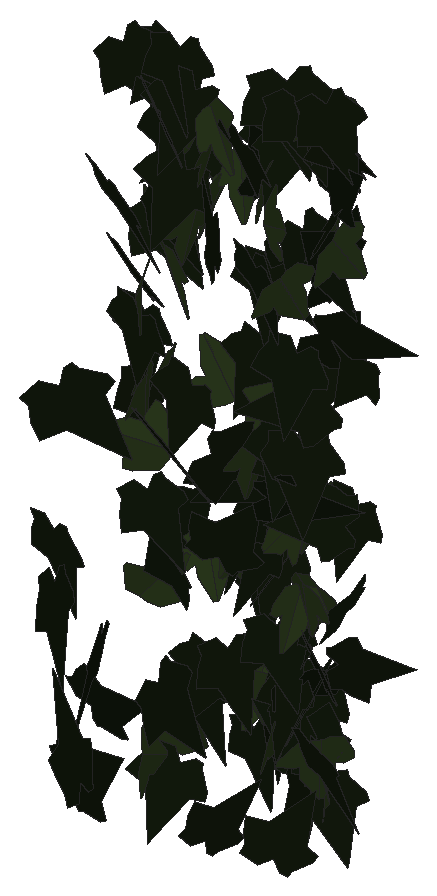
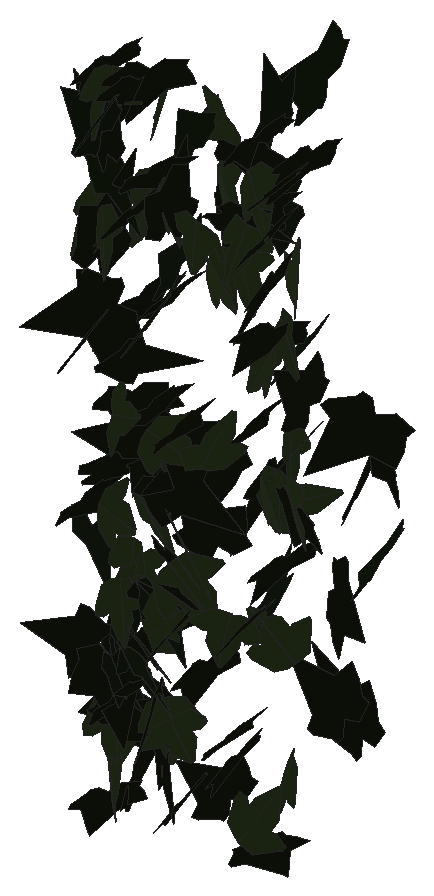
# SketchUp Ruby script. Lengths in inches.
U = 1.inch
M = Sketchup.active_model
def pt(a) = Geom::Point3d.new(a.map { |v| v * U })
def face(e, loops, mat)
  f = e.add_face(loops[0].map { |a| pt(a) })
  loops[1..].each { |l| e.add_face(l.map { |a| pt(a) }).erase! }
  f.material = f.back_material = mat if mat
  f
end
# faces: each face lists its corners as indices into pts; further lists are holes
def faces(e, pts, list, mat = nil) = list.each { |f| face(e, (f[0].is_a?(Array) ? f : [f]).map { |l| l.map { |i| pts[i] } }, mat) }
# xy, xz, yz: faces in a plane at the given z, y or x. An outline is a flat list of corners, or four numbers for a rectangle; further outlines are holes
def ring(l) = l.size == 4 ? [[l[0], l[1]], [l[2], l[1]], [l[2], l[3]], [l[0], l[3]]] : l.each_slice(2).to_a
def flat(e, list, mat, &to3) = list.each { |f| face(e, (f[0].is_a?(Array) ? f : [f]).map { |l| ring(l).map { |u, v| to3.(u, v) } }, mat) }
def xy(e, z, list, mat = nil) = flat(e, list, mat) { |x, y| [x, y, z] }
def xz(e, y, list, mat = nil) = flat(e, list, mat) { |x, z| [x, y, z] }
def yz(e, x, list, mat = nil) = flat(e, list, mat) { |y, z| [x, y, z] }
def lines(e, pts, list) = list.each { |a, b| e.add_line(pt(pts[a]), pt(pts[b])) }
# prism: a flat outline (further loops are holes) pulled along v
def prism(e, loops, v, mat = nil)
  f = face(e, loops, mat); d = Geom::Vector3d.new(v.map { |x| x * U })
  f.pushpull(f.normal.samedirection?(d) ? d.length : -d.length)
end
def box(e, o, s, mat = nil) = prism(e, [[o, [o[0] + s[0], o[1], o[2]], [o[0] + s[0], o[1] + s[1], o[2]], [o[0], o[1] + s[1], o[2]]]], [0, 0, s[2]], mat)
def at(x, y, z, deg = 0) = Geom::Transformation.translation(pt([x, y, z])) * Geom::Transformation.rotation(ORIGIN, Z_AXIS, deg.degrees)
def axes(o, x, y, z) = Geom::Transformation.new([*x, 0, *y, 0, *z, 0, *pt(o).to_a, 1])
def part(name) = M.definitions.add(name)
# library, detail: a bought-in or finely detailed component or shape, given as its bounding box
def library(name, o, s) = part(name).tap { |d| box(d.entities, o, s) }
def detail(e, o, s) = box(e.add_group.entities, o, s)
def put(e, d, t, mat = nil) = e.add_instance(d, t).tap { |i| i.material = mat if mat }
def group(e, t, mat = nil) = e.add_group.tap { |g| g.transformation = t; g.material = mat if mat }.entities
root = M.entities
M.materials.add("efeu1").color = [18, 25, 13]
M.materials.add("efeu2").color = [43, 57, 29]
c1 = part("ivyleaf_9")
p = [[1.54,2.16,1.25],[1.36,2.04,1.19],[-0.21,0.99,0.68],[-0.71,1.11,0.82],[-0.85,0.86,0.67],[-0.8,0.17,0.21],
  [-0.9,-0.01,0.1],[-0.67,-0.16,-0.02],[-0.08,-0.08,-0.05],[-0.03,-0.6,-0.4],[0.65,-0.88,-0.66],[0.83,-0.6,-0.49],
  [1.29,-0.42,-0.43],[1.8125,-0.07,-0.26],[1.21,0.44,0.15]]
faces(c1.entities,p,[[0,1,2,3,4,5,6,7,8,9,10,11,12,13,14]],"efeu1")
c2 = part("ivyleaf_10")
p = [[0,0.5,-0.03],[-0.0625,2.02,-0.43],[-0.19,2.01,-0.46],[-0.54,1.05,-0.29],[-0.52,0.625,-0.18],[-0.83,0.76,-0.28],
  [-1.16,0.64,-0.33],[-1.15,0.33,-0.24],[-0.77,-0.39,0.02],[-0.3,-0.51,0.16],[0.04,-0.48,0.23],[-0.02,2.01,-0.4375],
  [-0.06,2.01,-0.43],[0.04,-0.49,0.23],[0.67,-0.49,0.14],[1.38,0.36,-0.2],[1.375,0.51,-0.24],[0.81,0.65,-0.19],
  [0.62,0.59,-0.15],[0.6,1.09,-0.28],[0.5,1.23,-0.31]]
faces(c2.entities,p,[[0,1,2,3,4,5,6,7,8,9,10],[11,12,0,13,14,15,16,17,18,19,20]],"efeu2")
put(root,c1,axes([573.86,110.85,251.43],[-0.10242,-1.0928,1.02253],[0.0901,1.01856,1.09759],[-1.49388,0.13636,-0.00391]))
put(root,c1,axes([569.65,114.63,256.8],[-0.54052,-0.11963,-1.31812],[1.32353,-0.04442,-0.53871],[0.00412,-1.42395,0.12754]))
put(root,c1,axes([574.41,114.41,265.84],[1.30871,-0.42606,-0.11403],[-0.10734,0.03865,-1.37631],[0.42779,1.3131,0.00351]))
put(root,c1,axes([574.72,114.92,254.02],[0.53059,-0.75779,-0.98755],[-0.56809,0.80779,-0.92508],[1.10759,0.77733,-0.00139]))
put(root,c1,axes([570.54,117,273.96],[0.85935,-1.02214,0.66736],[0.41204,-0.52536,-1.33523],[1.14907,0.95281,-0.0203]))
put(root,c1,axes([567.85,118.16,245.98],[-0.09268,0.13273,1.43159],[0.9184,-1.09826,0.16129],[1.10617,0.92296,-0.01396]))
put(root,c1,axes([568.71,118.59,252.28],[-0.60556,0.38599,-1.26243],[1.0818,-0.65093,-0.71794],[-0.7566,-1.23965,-0.0161]))
put(root,c1,axes([565.42,119.9375,255.38],[0.49386,-1.12594,0.3271],[0.11112,-0.30839,-1.2293],[1.16722,0.50575,-0.02137]))
put(root,c1,axes([566.99,120.38,248.06],[0.15052,-0.24375,1.19736],[0.96166,-0.72066,-0.26759],[0.75386,0.96797,0.10228]))
put(root,c2,axes([568.71,121.3,266.89],[0.16425,-0.42355,-1.17811],[0.38377,-1.11397,0.454],[-1.19166,-0.41712,-0.01618]))
put(root,c1,axes([565.63,120.14,261.83],[-0.18279,-0.35002,-1.29683],[0.53968,1.17936,-0.39438],[1.23005,-0.56946,-0.01967]))
put(root,c2,axes([576.26,119.86,272.95],[-0.41112,0.4522,0.99052],[-0.61499,0.77729,-0.61011],[-0.89856,-0.7389,-0.03562]))
put(root,c1,axes([569.27,121.72,274.38],[0.04519,-0.46985,1.26714],[0.48066,-1.17936,-0.45444],[1.26308,0.46561,0.1276]))
put(root,c1,axes([575.69,120.79,244.23],[-0.56694,-0.08051,0.91684],[0.91933,0.00165,0.56862],[-0.04375,1.07797,0.06761]))
put(root,c1,axes([567.74,122.29,264.79],[0.10552,-1.03428,0.57558],[0.15766,-0.56044,-1.03596],[1.17311,0.16835,0.08745]))
put(root,c2,axes([575.56,121.5,269.35],[-0.42794,-0.97958,-0.5903],[0.21639,0.54954,-1.0688],[1.12303,-0.47916,-0.01899]))
put(root,c1,axes([571.68,121.63,243.26],[-0.10455,-0.20583,1.03103],[0.91019,0.5009,0.19229],[-0.52625,0.90722,0.12775]))
put(root,c1,axes([574.98,123.03,265.28],[-0.17149,-1.15961,0.09107],[-0.02017,-0.08908,-1.17221],[1.16301,-0.17254,-0.0069]))
put(root,c1,axes([571.78,121.875,269.02],[0.01584,-0.13978,1.28616],[-0.33463,1.24204,0.1391],[-1.2497,-0.33435,-0.02095]))
put(root,c2,axes([568.38,121.85,245.76],[0.28146,-0.57133,-1.07538],[-0.04694,1.09782,-0.59554],[1.21682,0.1745,0.22578]))
put(root,c2,axes([570.93,122.84,274.54],[0.74797,-0.10302,0.86127],[0.85496,-0.1045,-0.75498],[0.14649,1.13593,0.00866]))
put(root,c1,axes([569.05,123.47,271.24],[-0.42757,-1.09553,0.2771],[-0.08596,-0.26388,-1.17591],[1.12675,-0.43585,0.01544]))
put(root,c1,axes([568.19,123.6,253.67],[0.8151,-0.70151,-0.67063],[0.50656,-0.43949,1.07541],[-0.8278,-0.95968,-0.00226]))
put(root,c1,axes([571.42,122.73,255.33],[-0.47971,-0.1477,1.03329],[1.01018,-0.352,0.41866],[0.26279,1.08347,0.27687]))
put(root,c1,axes([571.84,123.63,273.36],[0.20991,-0.86177,0.88202],[0.43517,-0.78537,-0.87091],[1.15379,0.453,0.16801]))
put(root,c1,axes([569.1875,123.71,261.54],[-0.14884,-1.04741,0.50626],[0.001,-0.5105,-1.05589],[1.16334,-0.13356,0.06568]))
put(root,c2,axes([567.65,123.48,258.55],[0.27169,0.35664,1.17355],[-0.7659,-0.88952,0.44764],[0.95802,-0.81227,0.02506]))
put(root,c1,axes([574.03,123.66,260.89],[-0.18133,-1.13237,0.18259],[0.00393,-0.18547,-1.14632],[1.14699,-0.17838,0.03279]))
put(root,c1,axes([572.43,123.71,267.93],[0.47036,-1.01293,0.6329],[0.27772,-0.56881,-1.11676],[1.16166,0.54612,0.01073]))
put(root,c1,axes([575.05,123.39,261.03],[-0.54185,-0.95578,-0.49638],[0.20934,0.4516,-1.09807],[1.05645,-0.5797,-0.03701]))
put(root,c2,axes([567.47,122.92,261.53],[0.25977,-1.00547,-0.38903],[-0.01331,0.39714,-1.03533],[1.07803,0.24719,0.08096]))
put(root,c1,axes([573.98,122.7,258.71],[0.53554,0.54877,-1.05958],[0.72953,0.76849,0.76673],[0.94427,-0.90495,0.00857]))
put(root,c1,axes([575.41,123.5,247.73],[0.87827,-0.96416,0.25234],[0.15994,-0.19563,-1.30414],[0.98372,0.89262,-0.01325]))
put(root,c1,axes([567.32,123.42,256.34],[0.27879,-1.02264,-0.48464],[0.0414,0.50801,-1.04814],[1.13091,0.23351,0.15784]))
put(root,c2,axes([572.5625,123.64,260.12],[-0.0623,-1.19015,0.11543],[0.01415,-0.11631,-1.19161],[1.19565,-0.06064,0.02012]))
put(root,c2,axes([567.41,123.36,252.11],[-0.6393,-0.65848,0.65321],[0.46375,0.46012,0.91772],[-0.80325,0.78973,0.00996]))
put(root,c1,axes([571.07,123.69,250.41],[0.13657,-1.03082,-0.47157],[-0.092,0.46334,-1.03946],[1.12982,0.16234,-0.02764]))
put(root,c1,axes([575.51,124.1875,262.83],[-0.74346,-0.22338,0.9482],[-0.91351,-0.25443,-0.7762],[0.33836,-1.17775,-0.01216]))
put(root,c1,axes([571.19,122.68,259.72],[0.09394,0.19429,-1.26731],[-0.0812,1.26906,0.18854],[1.27955,0.06627,0.10501]))
put(root,c1,axes([568.97,124.12,274.48],[-1.00288,-0.57528,-0.28926],[0.24598,0.15249,-1.15613],[0.59507,-1.03257,-0.00959]))
put(root,c2,axes([569.18,123.85,269.16],[-0.02815,-1.12054,0.09049],[0.01426,-0.09087,-1.12077],[1.12409,-0.02691,0.01648]))
put(root,c1,axes([576.13,124.4375,257.51],[-0.64533,-0.05727,0.86038],[-0.72474,-0.54624,-0.57996],[0.4672,-0.92646,0.28876]))
put(root,c2,axes([574.29,124.05,253.76],[0.38268,0.90143,-0.42788],[-0.20699,-0.37659,-0.97849],[-0.97613,0.43326,0.03974]))
put(root,c1,axes([573.94,124.74,244.86],[0.24506,-0.3699,-1.06214],[0.84467,-0.65725,0.42378],[-0.74263,-0.86961,0.1315]))
put(root,c2,axes([569.88,124.12,272.83],[0.51281,-1.06387,0.03588],[0.00907,-0.03545,-1.18099],[1.06443,0.51284,-0.00722]))
put(root,c1,axes([575.7,124.06,276.17],[0.25693,-1.07445,-0.4585],[0.00744,0.47096,-1.09947],[1.16817,0.23332,0.10785]))
put(root,c1,axes([573.64,124.16,276.4],[-0.26043,-1.07272,-0.67278],[0.2523,0.62913,-1.10079],[1.24085,-0.35306,0.08262]))
put(root,c1,axes([576.21,123.93,271.5],[-0.8032,0.90095,-0.27324],[0.18572,-0.20049,-1.20699],[-0.92297,-0.82438,-0.00508]))
put(root,c1,axes([575.61,124.41,272.27],[-0.08914,0.04422,1.22627],[0.68922,-1.01542,0.08671],[1.01521,0.69324,0.0488]))
put(root,c1,axes([577.01,123.49,254.33],[-0.37109,0.9234,0.4039],[-0.18332,0.36138,-0.99464],[-0.99106,-0.41261,0.03275]))
put(root,c1,axes([567.77,124.65,243.75],[-0.59687,-0.94572,0.0103],[0.00597,-0.01595,-1.11824],[0.94576,-0.59674,0.01356]))
put(root,c2,axes([574.8,123.92,254.26],[-0.98483,0.37039,0.21185],[-0.212,0.03772,-1.05147],[-0.3703,-1.00665,0.03855]))
put(root,c1,axes([574.11,124.23,275.76],[0.01345,-1.01618,-0.58211],[0.09864,0.58106,-1.01208],[1.16694,-0.0374,0.09226]))
put(root,c1,axes([573.42,124.59,249.38],[-0.73409,-0.39739,-0.63975],[0.68526,0.01816,-0.7976],[0.31242,-0.97357,0.24625]))
put(root,c1,axes([572.92,124.43,251.75],[0.03625,-1.08694,-0.38663],[0.09147,0.38831,-1.08309],[1.15003,0.00337,0.09833]))
put(root,c2,axes([573.77,124.16,256.93],[0.8255,-0.44156,-0.64322],[-0.57974,0.27952,-0.93591],[0.52213,1.00849,-0.02223]))
put(root,c1,axes([565.63,124.07,275.4375],[0.34713,-0.861,-0.7275],[-0.06637,0.74428,-0.91253],[1.12524,0.30951,0.1706]))
put(root,c2,axes([575.17,124.27,247.24],[-0.74683,-0.98188,-0.02551],[0.01635,0.01961,-1.23363],[0.98208,-0.747,0.00114]))
put(root,c1,axes([572.34,124.7,258.67],[0.01461,-0.01696,-1.27934],[-0.7707,-1.02137,0.00473],[-1.02128,0.77053,-0.02188]))
put(root,c1,axes([567.8,124.72,275.67],[0.05963,-1.16155,-0.10993],[-0.00635,0.10975,-1.16308],[1.16672,0.05996,-0.00071]))
put(root,c2,axes([573.0625,123.91,247.6875],[0.43446,-0.91011,-0.76698],[-0.20039,0.74889,-1.00216],[1.1732,0.46495,0.11286]))
put(root,c1,axes([567.43,124.18,269.29],[0.62539,-0.87453,-0.61668],[-0.36027,0.50051,-1.07513],[1.00762,0.72174,-0.00166]))
put(root,c1,axes([572.28,124.69,255.37],[-1.0218,0.00735,-0.47474],[0.4745,-0.02459,-1.02164],[-0.01703,-1.12643,0.01921]))
put(root,c1,axes([568.95,125.25,248.43],[-0.28575,-0.962,0.52983],[0.03272,-0.55469,-0.98948],[1.09777,-0.23387,0.16741]))
put(root,c1,axes([572.05,125.09,267.15],[-0.07335,-1.08728,0.2572],[0.11437,-0.26371,-1.08217],[1.11142,-0.04462,0.12833]))
put(root,c1,axes([574.76,124.59,246.8],[-0.04284,0.23918,1.108],[-1.12702,0.10964,-0.06724],[-0.12128,-1.1034,0.23349]))
put(root,c1,axes([575.26,125.28,268.21],[0.21824,0.42013,1.3969],[-0.69211,-1.21352,0.4731],[1.28407,-0.72549,0.01758]))
put(root,c1,axes([574.33,124.42,269.93],[0.66415,-1.04697,-0.59352],[-0.16931,0.58987,-1.23],[1.19153,0.6674,0.15605]))
put(root,c1,axes([571.58,124.92,256.62],[-1.04282,0.24053,-0.72523],[0.70936,-0.15119,-1.07015],[-0.28392,-1.26118,-0.01002]))
put(root,c1,axes([574.99,124.7,250.06],[0.38323,-0.84721,0.88138],[-0.39535,0.78816,0.9295],[-1.15685,-0.55001,-0.02568]))
put(root,c1,axes([568.68,124.87,247.63],[0.41567,-1.03663,-0.23213],[-0.08862,0.21457,-1.11686],[1.0586,0.425,-0.00235]))
put(root,c1,axes([564.86,125.17,264.94],[0.42263,-0.62187,0.88306],[0.56717,-0.6792,-0.74976],[0.91914,0.70505,0.05661]))
put(root,c1,axes([568.83,125.3125,272.1],[-1.00169,-0.40724,0.33238],[-0.28176,-0.1879,-1.07935],[0.44377,-1.03853,0.06495]))
put(root,c2,axes([567.27,124.8,266.11],[-0.82288,0.68314,-0.46626],[0.35211,-0.3058,-1.06945],[-0.7484,-0.895,0.00951]))
put(root,c1,axes([565.5625,125.09,259.95],[-0.65793,-0.17528,-0.89599],[0.89176,0.11328,-0.67699],[0.19564,-1.10582,0.07267]))
put(root,c2,axes([575.96,124.35,269.97],[-0.14596,-0.98591,-0.71835],[0.32149,0.66681,-0.98049],[1.17673,-0.30446,0.17877]))
put(root,c1,axes([574.65,125.09,249.99],[-0.79662,0.56117,-0.67503],[0.51945,-0.43348,-0.97337],[-0.70764,-0.94993,0.0454]))
put(root,c1,axes([566.9,125.53,271.7],[0.05803,-1.11771,0.36298],[0.05768,-0.36028,-1.1186],[1.17376,0.07296,0.03703]))
put(root,c1,axes([575.35,125.77,273.69],[-0.37791,-0.39798,1.02082],[-0.1718,-1.04495,-0.47099],[1.0821,-0.30489,0.28173]))
put(root,c2,axes([572.01,125.13,271.67],[0.48291,-1.0045,0.19161],[0.08156,-0.17339,-1.11455],[1.01935,0.48974,-0.00159]))
put(root,c2,axes([575.24,124.59,275.52],[-0.43895,-0.96935,-0.44434],[0.17515,0.40845,-1.06408],[1.05186,-0.47253,-0.00825]))
put(root,c2,axes([572.01,125.66,261.09],[-0.35559,-0.66207,0.84033],[-0.11336,-0.85723,-0.72336],[1.06379,-0.31266,0.20381]))
put(root,c2,axes([567.85,125.16,244.69],[-0.97559,0.00171,-0.57933],[-0.57857,-0.06107,0.97413],[-0.02972,1.13299,0.05338]))
put(root,c2,axes([571.1,125.46,255.06],[-0.54873,-0.88,0.71355],[-0.38531,-0.60063,-1.03704],[1.06541,-0.67046,-0.00754]))
put(root,c1,axes([575.06,125.5,273.82],[0.36367,-0.56307,0.97952],[0.66033,-0.72904,-0.66425],[0.91677,0.74848,0.08988]))
put(root,c1,axes([565.3,125.63,262.67],[0.1953,-1.08259,0.29529],[0.08669,-0.28428,-1.09955],[1.11879,0.21101,0.03365]))
put(root,c2,axes([568.26,124.7,271.49],[-0.25024,-0.9226,-0.63681],[0.21687,0.60032,-0.95495],[1.09986,-0.32828,0.04341]))
put(root,c2,axes([567.43,125.32,273.93],[0.14361,-1.16815,0.11398],[0.01736,-0.11271,-1.17694],[1.17357,0.14461,0.00347]))
put(root,c2,axes([566.48,124.77,267.44],[-0.4563,0.15198,1.0031],[-0.94617,0.33321,-0.48089],[-0.36616,-1.05043,-0.00742]))
put(root,c2,axes([571.85,125.19,248.67],[-0.8731,-0.55762,0.13382],[-0.10318,-0.08703,-1.03583],[0.5641,-0.879,0.01767]))
put(root,c2,axes([565.46,125.375,260.57],[0.57714,-0.9261,-0.01061],[-0.01749,0.0016,-1.09113],[0.926,0.57724,-0.014]))
put(root,c1,axes([572.23,125.93,273.0625],[-0.40663,-1.0623,0.14187],[0.05658,-0.17281,-1.13176],[1.07023,-0.39447,0.11374]))
put(root,c1,axes([566.16,126.18,274.28],[-0.41669,-0.81394,0.69371],[-0.02224,-0.73775,-0.87897],[1.06922,-0.33255,0.25206]))
put(root,c1,axes([571.41,125.66,271],[0.2168,0.63503,0.99661],[-0.57272,-0.82983,0.65335],[1.03368,-0.59297,0.15297]))
put(root,c2,axes([569.03,125.7,269.72],[0.31727,-0.99417,0.40773],[0.09286,-0.39817,-1.04313],[1.07051,0.32919,-0.03035]))
put(root,c1,axes([575.73,126.24,263.93],[-0.17325,-0.7848,0.82455],[-0.03246,-0.8303,-0.79709],[1.13787,-0.14318,0.1028]))
put(root,c2,axes([568.71,125.25,253.76],[0.94799,0.56567,0.28702],[0.24069,0.15674,-1.10388],[-0.58688,0.97801,0.01091]))
put(root,c1,axes([566.44,125.33,267.76],[0.08701,-0.92088,-0.7029],[0.22036,0.70517,-0.89658],[1.13734,-0.06618,0.22748]))
put(root,c2,axes([574.16,126.05,257.23],[0.21753,-0.74025,0.81435],[0.2344,-0.77989,-0.77155],[1.07526,0.31976,0.00345]))
put(root,c1,axes([575.04,124.67,265.5625],[0.16165,0.40591,-1.21053],[0.52749,1.08996,0.43591],[1.16271,-0.55092,-0.02947]))
put(root,c1,axes([572.45,124.9,246.86],[0.10036,0.10696,-1.20825],[-1.20426,0.15384,-0.08641],[0.14512,1.20261,0.11852]))
put(root,c1,axes([573.15,125.76,251.97],[-0.93392,0.13526,-0.46488],[0.4418,-0.1751,-0.93849],[-0.19805,-1.02843,0.09865]))
put(root,c1,axes([571.06,126.02,252.8],[0.14072,-1.01076,0.2547],[0.01387,-0.25517,-1.0203],[1.04227,0.13986,-0.0208]))
put(root,c2,axes([570.07,125.52,271.02],[1.08635,-0.06274,0.33696],[0.34083,0.07925,-1.08406],[0.03627,1.13464,0.09435]))
put(root,c1,axes([573.93,126.15,248.78],[-0.23756,-0.97421,0.30432],[-0.07642,-0.2946,-1.00275],[1.01777,-0.24951,-0.00426]))
put(root,c2,axes([573.86,126.01,244.47],[-0.28847,0.16868,1.14152],[0.96824,-0.6047,0.33404],[0.62772,1.01025,0.00935]))
put(root,c2,axes([573.74,126.14,261.75],[-0.22206,0.56884,-0.97487],[-0.05233,-0.99768,-0.57023],[-1.12748,-0.06573,0.21847]))
put(root,c1,axes([572.34,125.27,253.93],[-0.53079,0.94881,-0.14514],[0.07078,-0.12671,-1.08718],[-0.95723,-0.53549,0.00009]))
put(root,c1,axes([575.42,126.17,257.31],[-0.18607,-1.05331,0.25953],[-0.0276,-0.25864,-1.06948],[1.08446,-0.18731,0.01731]))
put(root,c1,axes([573.57,125.44,250.89],[-0.84345,0.63927,-0.03384],[0.02514,-0.02285,-1.05833],[-0.63967,-0.84382,0.00302]))
put(root,c2,axes([569.5625,125.51,260.95],[0.40858,1.07105,0.31506],[-0.16849,-0.27249,1.14486],[1.10364,-0.43812,0.05815]))
put(root,c1,axes([572.58,124.875,248.99],[0.35345,-0.02431,-0.98557],[-0.8286,0.55999,-0.31097],[0.53419,0.88469,0.16975]))
put(root,c2,axes([571.08,125.73,248.49],[0.58768,0.84094,-0.38065],[-0.20166,-0.32338,-1.02576],[-0.90078,0.62103,-0.01869]))
put(root,c2,axes([566.36,125.86,260.91],[0.45825,-0.95431,0.27283],[0.15406,-0.22847,-1.05793],[0.98052,0.4819,0.03872]))
put(root,c2,axes([571.42,126.39,253.09],[-0.27918,-0.24398,-1.07687],[-0.40514,-1.01065,0.33401],[-1.02715,0.46494,0.16095]))
put(root,c1,axes([571.74,125.34,267.4],[0.77296,-0.68624,-0.53505],[-0.29705,0.46457,-1.02499],[0.8179,0.81727,0.13338]))
put(root,c1,axes([567.66,126.48,253.91],[-0.41198,-0.54548,0.85973],[-0.13381,-0.89039,-0.62906],[1.00934,-0.34069,0.26752]))
put(root,c1,axes([571.875,125.97,254.41],[-0.80084,-0.56478,-0.39797],[0.3356,0.21455,-0.97982],[0.60393,-0.86815,0.01676]))
put(root,c1,axes([574.59,125.33,250.01],[0.13384,1.10095,-0.43754],[-0.05559,-0.434,-1.10905],[-1.1834,0.1449,0.00262]))
put(root,c1,axes([570.52,126.47,262.3125],[-0.24392,-0.97099,0.50201],[-0.0511,-0.50367,-0.99902],[1.0919,-0.24048,0.06539]))
put(root,c2,axes([574.78,125.53,269.8125],[0.30192,-1.02699,-0.35884],[-0.01961,0.36721,-1.06743],[1.0877,0.29169,0.08036]))
put(root,c2,axes([574.12,125.49,253.32],[-0.95828,0.06982,0.44465],[-0.44128,0.06024,-0.96048],[-0.08864,-1.05469,-0.02542]))
put(root,c1,axes([570.42,126.09,245.57],[0.34647,-1.05732,0.04467],[0.01334,-0.04263,-1.11264],[1.05818,0.34673,-0.0006]))
put(root,c1,axes([575.38,125.35,250.62],[0.5942,0.26436,-0.83644],[0.49991,0.72812,0.58525],[0.72084,-0.72287,0.28361]))
put(root,c1,axes([574.23,125.97,244.5],[-0.12121,-0.97443,-0.49667],[0.15847,0.47879,-0.97802],[1.08216,-0.17925,0.08759]))
